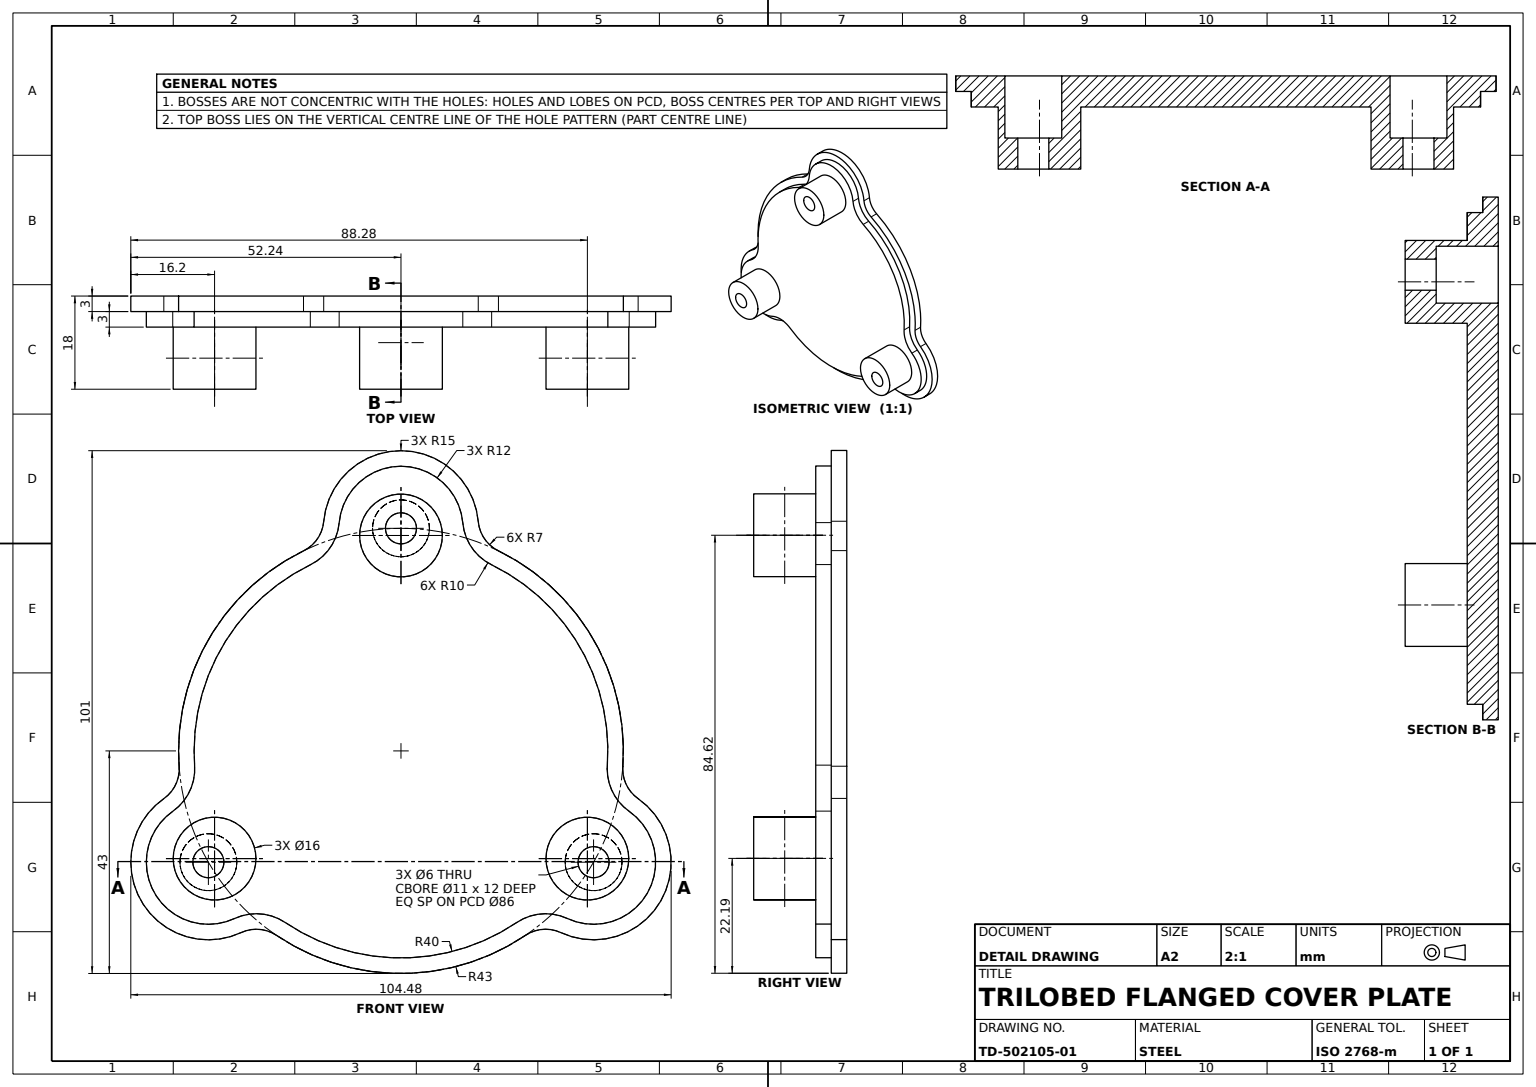
ISO-10303-21;
HEADER;
FILE_DESCRIPTION((''),'2;1');
FILE_NAME('','',(''),(''),'','','');
FILE_SCHEMA(('AUTOMOTIVE_DESIGN'));
ENDSEC;
DATA;
#1=APPLICATION_CONTEXT('');
#2=PRODUCT_CONTEXT('',#1,'mechanical');
#3=PRODUCT('','','',(#2));
#4=PRODUCT_DEFINITION_FORMATION('','',#3);
#5=PRODUCT_DEFINITION_CONTEXT('',#1,'design');
#6=PRODUCT_DEFINITION('','',#4,#5);
#7=PRODUCT_DEFINITION_SHAPE('','',#6);
#8=(LENGTH_UNIT()NAMED_UNIT(*)SI_UNIT(.MILLI.,.METRE.));
#9=(NAMED_UNIT(*)PLANE_ANGLE_UNIT()SI_UNIT($,.RADIAN.));
#10=(NAMED_UNIT(*)SI_UNIT($,.STERADIAN.)SOLID_ANGLE_UNIT());
#11=UNCERTAINTY_MEASURE_WITH_UNIT(LENGTH_MEASURE(1.E-05),#8,'distance_accuracy_value','');
#12=(GEOMETRIC_REPRESENTATION_CONTEXT(3)GLOBAL_UNCERTAINTY_ASSIGNED_CONTEXT((#11))GLOBAL_UNIT_ASSIGNED_CONTEXT((#8,#9,#10))REPRESENTATION_CONTEXT('',''));
#13=CARTESIAN_POINT('',(24.048805,-35.646248,-3.));
#14=VERTEX_POINT('',#13);
#15=CARTESIAN_POINT('',(24.048805,-35.646248,0.));
#16=VERTEX_POINT('',#15);
#17=DIRECTION('',(0.,0.,1.));
#18=VECTOR('',#17,1000.);
#19=LINE('',#13,#18);
#20=EDGE_CURVE('',#14,#16,#19,.T.);
#21=ORIENTED_EDGE('',*,*,#20,.T.);
#22=CARTESIAN_POINT('',(-24.048805,-35.646248,0.));
#23=VERTEX_POINT('',#22);
#24=CARTESIAN_POINT('',(0.,0.,0.));
#25=DIRECTION('',(1.,0.,0.));
#26=AXIS2_PLACEMENT_3D('',#24,#17,#25);
#27=CIRCLE('',#26,43.);
#28=EDGE_CURVE('',#23,#16,#27,.T.);
#29=ORIENTED_EDGE('',*,*,#28,.F.);
#30=CARTESIAN_POINT('',(-24.048805,-35.646248,-3.));
#31=VERTEX_POINT('',#30);
#32=LINE('',#30,#18);
#33=EDGE_CURVE('',#31,#23,#32,.T.);
#34=ORIENTED_EDGE('',*,*,#33,.F.);
#35=CARTESIAN_POINT('',(0.,0.,-3.));
#36=AXIS2_PLACEMENT_3D('',#35,#17,#25);
#37=CIRCLE('',#36,43.);
#38=EDGE_CURVE('',#31,#14,#37,.T.);
#39=ORIENTED_EDGE('',*,*,#38,.T.);
#40=EDGE_LOOP('',(#21,#29,#34,#39));
#41=FACE_OUTER_BOUND('',#40,.T.);
#42=CYLINDRICAL_SURFACE('',#36,43.);
#43=ADVANCED_FACE('',(#41),#42,.T.);
#44=CARTESIAN_POINT('',(-28.042979,-20.809424,-18.));
#45=VERTEX_POINT('',#44);
#46=CARTESIAN_POINT('',(-44.042979,-20.809424,-18.));
#47=VERTEX_POINT('',#46);
#48=CARTESIAN_POINT('',(-36.042979,-20.809424,-18.));
#49=DIRECTION('',(0.,0.,-1.));
#50=DIRECTION('',(-1.,0.,0.));
#51=AXIS2_PLACEMENT_3D('',#48,#49,#50);
#52=CIRCLE('',#51,8.);
#53=EDGE_CURVE('',#45,#47,#52,.T.);
#54=ORIENTED_EDGE('',*,*,#53,.T.);
#55=EDGE_CURVE('',#47,#45,#52,.T.);
#56=ORIENTED_EDGE('',*,*,#55,.T.);
#57=EDGE_LOOP('',(#54,#56));
#58=FACE_OUTER_BOUND('',#57,.T.);
#59=CARTESIAN_POINT('',(-34.239092,-21.5,-18.));
#60=VERTEX_POINT('',#59);
#61=CARTESIAN_POINT('',(-40.239092,-21.5,-18.));
#62=VERTEX_POINT('',#61);
#63=CARTESIAN_POINT('',(-37.239092,-21.5,-18.));
#64=AXIS2_PLACEMENT_3D('',#63,#49,#50);
#65=CIRCLE('',#64,3.);
#66=EDGE_CURVE('',#60,#62,#65,.T.);
#67=ORIENTED_EDGE('',*,*,#66,.F.);
#68=EDGE_CURVE('',#62,#60,#65,.T.);
#69=ORIENTED_EDGE('',*,*,#68,.F.);
#70=EDGE_LOOP('',(#67,#69));
#71=FACE_BOUND('',#70,.T.);
#72=PLANE('',#51);
#73=ADVANCED_FACE('',(#58,#71),#72,.T.);
#74=CARTESIAN_POINT('',(-44.042979,-20.809424,-6.));
#75=VERTEX_POINT('',#74);
#76=CARTESIAN_POINT('',(-28.042979,-20.809424,-6.));
#77=VERTEX_POINT('',#76);
#78=CARTESIAN_POINT('',(-36.042979,-20.809424,-6.));
#79=AXIS2_PLACEMENT_3D('',#78,#49,#50);
#80=CIRCLE('',#79,8.);
#81=EDGE_CURVE('',#75,#77,#80,.T.);
#82=ORIENTED_EDGE('',*,*,#81,.T.);
#83=LINE('',#44,#18);
#84=EDGE_CURVE('',#45,#77,#83,.T.);
#85=ORIENTED_EDGE('',*,*,#84,.F.);
#86=ORIENTED_EDGE('',*,*,#55,.F.);
#87=LINE('',#46,#18);
#88=EDGE_CURVE('',#47,#75,#87,.T.);
#89=ORIENTED_EDGE('',*,*,#88,.T.);
#90=EDGE_LOOP('',(#82,#85,#86,#89));
#91=FACE_OUTER_BOUND('',#90,.T.);
#92=AXIS2_PLACEMENT_3D('',#48,#17,#25);
#93=CYLINDRICAL_SURFACE('',#92,8.);
#94=ADVANCED_FACE('',(#91),#93,.T.);
#95=CARTESIAN_POINT('',(22.370982,-33.1593,-6.));
#96=VERTEX_POINT('',#95);
#97=CARTESIAN_POINT('',(-22.370982,-33.1593,-6.));
#98=VERTEX_POINT('',#97);
#99=CARTESIAN_POINT('',(0.,0.,-6.));
#100=AXIS2_PLACEMENT_3D('',#99,#49,#50);
#101=CIRCLE('',#100,40.);
#102=EDGE_CURVE('',#96,#98,#101,.T.);
#103=ORIENTED_EDGE('',*,*,#102,.T.);
#104=CARTESIAN_POINT('',(-32.179802,-32.381341,-6.));
#105=VERTEX_POINT('',#104);
#106=CARTESIAN_POINT('',(-27.963727,-41.449125,-6.));
#107=AXIS2_PLACEMENT_3D('',#106,#17,#50);
#108=CIRCLE('',#107,10.);
#109=EDGE_CURVE('',#98,#105,#108,.T.);
#110=ORIENTED_EDGE('',*,*,#109,.T.);
#111=CARTESIAN_POINT('',(-44.132965,-11.677856,-6.));
#112=VERTEX_POINT('',#111);
#113=CARTESIAN_POINT('',(-37.239092,-21.5,-6.));
#114=AXIS2_PLACEMENT_3D('',#113,#49,#50);
#115=CIRCLE('',#114,12.);
#116=EDGE_CURVE('',#105,#112,#115,.T.);
#117=ORIENTED_EDGE('',*,*,#116,.T.);
#118=CARTESIAN_POINT('',(-39.877859,-3.492735,-6.));
#119=VERTEX_POINT('',#118);
#120=CARTESIAN_POINT('',(-49.877859,-3.492735,-6.));
#121=AXIS2_PLACEMENT_3D('',#120,#17,#50);
#122=CIRCLE('',#121,10.);
#123=EDGE_CURVE('',#112,#119,#122,.T.);
#124=ORIENTED_EDGE('',*,*,#123,.T.);
#125=CARTESIAN_POINT('',(-39.902287,-2.794188,-6.));
#126=VERTEX_POINT('',#125);
#127=EDGE_CURVE('',#119,#126,#122,.T.);
#128=ORIENTED_EDGE('',*,*,#127,.T.);
#129=CARTESIAN_POINT('',(-17.531306,35.953488,-6.));
#130=VERTEX_POINT('',#129);
#131=EDGE_CURVE('',#126,#130,#101,.T.);
#132=ORIENTED_EDGE('',*,*,#131,.T.);
#133=CARTESIAN_POINT('',(-11.953163,44.059197,-6.));
#134=VERTEX_POINT('',#133);
#135=CARTESIAN_POINT('',(-21.914132,44.94186,-6.));
#136=AXIS2_PLACEMENT_3D('',#135,#17,#50);
#137=CIRCLE('',#136,10.);
#138=EDGE_CURVE('',#130,#134,#137,.T.);
#139=ORIENTED_EDGE('',*,*,#138,.T.);
#140=CARTESIAN_POINT('',(11.953163,44.059197,-6.));
#141=VERTEX_POINT('',#140);
#142=CARTESIAN_POINT('',(0.,43.,-6.));
#143=AXIS2_PLACEMENT_3D('',#142,#49,#50);
#144=CIRCLE('',#143,12.);
#145=EDGE_CURVE('',#134,#141,#144,.T.);
#146=ORIENTED_EDGE('',*,*,#145,.T.);
#147=CARTESIAN_POINT('',(17.531306,35.953488,-6.));
#148=VERTEX_POINT('',#147);
#149=CARTESIAN_POINT('',(21.914132,44.94186,-6.));
#150=AXIS2_PLACEMENT_3D('',#149,#17,#50);
#151=CIRCLE('',#150,10.);
#152=EDGE_CURVE('',#141,#148,#151,.T.);
#153=ORIENTED_EDGE('',*,*,#152,.T.);
#154=CARTESIAN_POINT('',(40.,0.,-6.));
#155=VERTEX_POINT('',#154);
#156=EDGE_CURVE('',#148,#155,#101,.T.);
#157=ORIENTED_EDGE('',*,*,#156,.T.);
#158=CARTESIAN_POINT('',(39.902287,-2.794188,-6.));
#159=VERTEX_POINT('',#158);
#160=EDGE_CURVE('',#155,#159,#101,.T.);
#161=ORIENTED_EDGE('',*,*,#160,.T.);
#162=CARTESIAN_POINT('',(44.132965,-11.677856,-6.));
#163=VERTEX_POINT('',#162);
#164=CARTESIAN_POINT('',(49.877859,-3.492735,-6.));
#165=AXIS2_PLACEMENT_3D('',#164,#17,#50);
#166=CIRCLE('',#165,10.);
#167=EDGE_CURVE('',#159,#163,#166,.T.);
#168=ORIENTED_EDGE('',*,*,#167,.T.);
#169=CARTESIAN_POINT('',(49.239092,-21.5,-6.));
#170=VERTEX_POINT('',#169);
#171=CARTESIAN_POINT('',(37.239092,-21.5,-6.));
#172=AXIS2_PLACEMENT_3D('',#171,#49,#50);
#173=CIRCLE('',#172,12.);
#174=EDGE_CURVE('',#163,#170,#173,.T.);
#175=ORIENTED_EDGE('',*,*,#174,.T.);
#176=CARTESIAN_POINT('',(32.179802,-32.381341,-6.));
#177=VERTEX_POINT('',#176);
#178=EDGE_CURVE('',#170,#177,#173,.T.);
#179=ORIENTED_EDGE('',*,*,#178,.T.);
#180=CARTESIAN_POINT('',(27.963727,-41.449125,-6.));
#181=AXIS2_PLACEMENT_3D('',#180,#17,#50);
#182=CIRCLE('',#181,10.);
#183=EDGE_CURVE('',#177,#96,#182,.T.);
#184=ORIENTED_EDGE('',*,*,#183,.T.);
#185=EDGE_LOOP('',(#103,#110,#117,#124,#128,#132,#139,#146,#153,#157,#161,#168,#175,#179,#184));
#186=FACE_OUTER_BOUND('',#185,.T.);
#187=CARTESIAN_POINT('',(44.042979,-20.809424,-6.));
#188=VERTEX_POINT('',#187);
#189=CARTESIAN_POINT('',(28.042979,-20.809424,-6.));
#190=VERTEX_POINT('',#189);
#191=CARTESIAN_POINT('',(36.042979,-20.809424,-6.));
#192=AXIS2_PLACEMENT_3D('',#191,#49,#50);
#193=CIRCLE('',#192,8.);
#194=EDGE_CURVE('',#188,#190,#193,.T.);
#195=ORIENTED_EDGE('',*,*,#194,.F.);
#196=EDGE_CURVE('',#190,#188,#193,.T.);
#197=ORIENTED_EDGE('',*,*,#196,.F.);
#198=EDGE_LOOP('',(#195,#197));
#199=FACE_BOUND('',#198,.T.);
#200=CARTESIAN_POINT('',(8.,41.618847,-6.));
#201=VERTEX_POINT('',#200);
#202=CARTESIAN_POINT('',(-8.,41.618847,-6.));
#203=VERTEX_POINT('',#202);
#204=CARTESIAN_POINT('',(0.,41.618847,-6.));
#205=AXIS2_PLACEMENT_3D('',#204,#49,#50);
#206=CIRCLE('',#205,8.);
#207=EDGE_CURVE('',#201,#203,#206,.T.);
#208=ORIENTED_EDGE('',*,*,#207,.F.);
#209=EDGE_CURVE('',#203,#201,#206,.T.);
#210=ORIENTED_EDGE('',*,*,#209,.F.);
#211=EDGE_LOOP('',(#208,#210));
#212=FACE_BOUND('',#211,.T.);
#213=ORIENTED_EDGE('',*,*,#81,.F.);
#214=EDGE_CURVE('',#77,#75,#80,.T.);
#215=ORIENTED_EDGE('',*,*,#214,.F.);
#216=EDGE_LOOP('',(#213,#215));
#217=FACE_BOUND('',#216,.T.);
#218=CARTESIAN_POINT('',(10.957066,43.97093,-6.));
#219=AXIS2_PLACEMENT_3D('',#218,#49,#50);
#220=PLANE('',#219);
#221=ADVANCED_FACE('',(#186,#199,#212,#217),#220,.T.);
#222=CARTESIAN_POINT('',(-8.,41.618847,-18.));
#223=VERTEX_POINT('',#222);
#224=CARTESIAN_POINT('',(8.,41.618847,-18.));
#225=VERTEX_POINT('',#224);
#226=CARTESIAN_POINT('',(0.,41.618847,-18.));
#227=AXIS2_PLACEMENT_3D('',#226,#49,#50);
#228=CIRCLE('',#227,8.);
#229=EDGE_CURVE('',#223,#225,#228,.T.);
#230=ORIENTED_EDGE('',*,*,#229,.F.);
#231=LINE('',#222,#18);
#232=EDGE_CURVE('',#223,#203,#231,.T.);
#233=ORIENTED_EDGE('',*,*,#232,.T.);
#234=ORIENTED_EDGE('',*,*,#209,.T.);
#235=LINE('',#224,#18);
#236=EDGE_CURVE('',#225,#201,#235,.T.);
#237=ORIENTED_EDGE('',*,*,#236,.F.);
#238=EDGE_LOOP('',(#230,#233,#234,#237));
#239=FACE_OUTER_BOUND('',#238,.T.);
#240=AXIS2_PLACEMENT_3D('',#226,#17,#25);
#241=CYLINDRICAL_SURFACE('',#240,8.);
#242=ADVANCED_FACE('',(#239),#241,.T.);
#243=CARTESIAN_POINT('',(-30.91498,-35.101676,-3.));
#244=VERTEX_POINT('',#243);
#245=CARTESIAN_POINT('',(-30.91498,-35.101676,0.));
#246=VERTEX_POINT('',#245);
#247=LINE('',#243,#18);
#248=EDGE_CURVE('',#244,#246,#247,.T.);
#249=ORIENTED_EDGE('',*,*,#248,.F.);
#250=CARTESIAN_POINT('',(-27.963727,-41.449125,-3.));
#251=AXIS2_PLACEMENT_3D('',#250,#49,#50);
#252=CIRCLE('',#251,7.);
#253=EDGE_CURVE('',#244,#31,#252,.T.);
#254=ORIENTED_EDGE('',*,*,#253,.T.);
#255=ORIENTED_EDGE('',*,*,#33,.T.);
#256=CARTESIAN_POINT('',(-27.963727,-41.449125,0.));
#257=AXIS2_PLACEMENT_3D('',#256,#49,#50);
#258=CIRCLE('',#257,7.);
#259=EDGE_CURVE('',#246,#23,#258,.T.);
#260=ORIENTED_EDGE('',*,*,#259,.F.);
#261=EDGE_LOOP('',(#249,#254,#255,#260));
#262=FACE_OUTER_BOUND('',#261,.T.);
#263=AXIS2_PLACEMENT_3D('',#250,#17,#25);
#264=CYLINDRICAL_SURFACE('',#263,7.);
#265=ADVANCED_FACE('',(#262),#264,.F.);
#266=CARTESIAN_POINT('',(-5.5,43.,-12.));
#267=VERTEX_POINT('',#266);
#268=CARTESIAN_POINT('',(5.5,43.,-12.));
#269=VERTEX_POINT('',#268);
#270=CARTESIAN_POINT('',(0.,43.,-12.));
#271=AXIS2_PLACEMENT_3D('',#270,#17,#25);
#272=CIRCLE('',#271,5.5);
#273=EDGE_CURVE('',#267,#269,#272,.T.);
#274=ORIENTED_EDGE('',*,*,#273,.F.);
#275=CARTESIAN_POINT('',(-5.5,43.,0.));
#276=VERTEX_POINT('',#275);
#277=LINE('',#266,#18);
#278=EDGE_CURVE('',#267,#276,#277,.T.);
#279=ORIENTED_EDGE('',*,*,#278,.T.);
#280=CARTESIAN_POINT('',(5.5,43.,0.));
#281=VERTEX_POINT('',#280);
#282=CARTESIAN_POINT('',(0.,43.,0.));
#283=AXIS2_PLACEMENT_3D('',#282,#17,#25);
#284=CIRCLE('',#283,5.5);
#285=EDGE_CURVE('',#276,#281,#284,.T.);
#286=ORIENTED_EDGE('',*,*,#285,.T.);
#287=LINE('',#268,#18);
#288=EDGE_CURVE('',#269,#281,#287,.T.);
#289=ORIENTED_EDGE('',*,*,#288,.F.);
#290=EDGE_LOOP('',(#274,#279,#286,#289));
#291=FACE_OUTER_BOUND('',#290,.T.);
#292=CYLINDRICAL_SURFACE('',#271,5.5);
#293=ADVANCED_FACE('',(#291),#292,.F.);
#294=ORIENTED_EDGE('',*,*,#288,.T.);
#295=EDGE_CURVE('',#281,#276,#284,.T.);
#296=ORIENTED_EDGE('',*,*,#295,.T.);
#297=ORIENTED_EDGE('',*,*,#278,.F.);
#298=EDGE_CURVE('',#269,#267,#272,.T.);
#299=ORIENTED_EDGE('',*,*,#298,.F.);
#300=EDGE_LOOP('',(#294,#296,#297,#299));
#301=FACE_OUTER_BOUND('',#300,.T.);
#302=ADVANCED_FACE('',(#301),#292,.F.);
#303=CARTESIAN_POINT('',(-42.739092,-21.5,-12.));
#304=VERTEX_POINT('',#303);
#305=CARTESIAN_POINT('',(-42.739092,-21.5,0.));
#306=VERTEX_POINT('',#305);
#307=LINE('',#303,#18);
#308=EDGE_CURVE('',#304,#306,#307,.T.);
#309=ORIENTED_EDGE('',*,*,#308,.T.);
#310=CARTESIAN_POINT('',(-31.739092,-21.5,0.));
#311=VERTEX_POINT('',#310);
#312=CARTESIAN_POINT('',(-37.239092,-21.5,0.));
#313=AXIS2_PLACEMENT_3D('',#312,#17,#25);
#314=CIRCLE('',#313,5.5);
#315=EDGE_CURVE('',#306,#311,#314,.T.);
#316=ORIENTED_EDGE('',*,*,#315,.T.);
#317=CARTESIAN_POINT('',(-31.739092,-21.5,-12.));
#318=VERTEX_POINT('',#317);
#319=LINE('',#317,#18);
#320=EDGE_CURVE('',#318,#311,#319,.T.);
#321=ORIENTED_EDGE('',*,*,#320,.F.);
#322=CARTESIAN_POINT('',(-37.239092,-21.5,-12.));
#323=AXIS2_PLACEMENT_3D('',#322,#17,#25);
#324=CIRCLE('',#323,5.5);
#325=EDGE_CURVE('',#304,#318,#324,.T.);
#326=ORIENTED_EDGE('',*,*,#325,.F.);
#327=EDGE_LOOP('',(#309,#316,#321,#326));
#328=FACE_OUTER_BOUND('',#327,.T.);
#329=CYLINDRICAL_SURFACE('',#323,5.5);
#330=ADVANCED_FACE('',(#328),#329,.F.);
#331=CARTESIAN_POINT('',(-17.531306,35.953488,-3.));
#332=VERTEX_POINT('',#331);
#333=LINE('',#129,#18);
#334=EDGE_CURVE('',#130,#332,#333,.T.);
#335=ORIENTED_EDGE('',*,*,#334,.T.);
#336=CARTESIAN_POINT('',(-11.953163,44.059197,-3.));
#337=VERTEX_POINT('',#336);
#338=CARTESIAN_POINT('',(-21.914132,44.94186,-3.));
#339=AXIS2_PLACEMENT_3D('',#338,#17,#50);
#340=CIRCLE('',#339,10.);
#341=EDGE_CURVE('',#332,#337,#340,.T.);
#342=ORIENTED_EDGE('',*,*,#341,.T.);
#343=LINE('',#133,#18);
#344=EDGE_CURVE('',#134,#337,#343,.T.);
#345=ORIENTED_EDGE('',*,*,#344,.F.);
#346=ORIENTED_EDGE('',*,*,#138,.F.);
#347=EDGE_LOOP('',(#335,#342,#345,#346));
#348=FACE_OUTER_BOUND('',#347,.T.);
#349=AXIS2_PLACEMENT_3D('',#135,#17,#25);
#350=CYLINDRICAL_SURFACE('',#349,10.);
#351=ADVANCED_FACE('',(#348),#350,.F.);
#352=CARTESIAN_POINT('',(-44.132965,-11.677856,-3.));
#353=VERTEX_POINT('',#352);
#354=CARTESIAN_POINT('',(-39.877859,-3.492735,-3.));
#355=VERTEX_POINT('',#354);
#356=CARTESIAN_POINT('',(-49.877859,-3.492735,-3.));
#357=AXIS2_PLACEMENT_3D('',#356,#17,#50);
#358=CIRCLE('',#357,10.);
#359=EDGE_CURVE('',#353,#355,#358,.T.);
#360=ORIENTED_EDGE('',*,*,#359,.T.);
#361=LINE('',#118,#18);
#362=EDGE_CURVE('',#119,#355,#361,.T.);
#363=ORIENTED_EDGE('',*,*,#362,.F.);
#364=ORIENTED_EDGE('',*,*,#123,.F.);
#365=LINE('',#111,#18);
#366=EDGE_CURVE('',#112,#353,#365,.T.);
#367=ORIENTED_EDGE('',*,*,#366,.T.);
#368=EDGE_LOOP('',(#360,#363,#364,#367));
#369=FACE_OUTER_BOUND('',#368,.T.);
#370=AXIS2_PLACEMENT_3D('',#120,#17,#25);
#371=CYLINDRICAL_SURFACE('',#370,10.);
#372=ADVANCED_FACE('',(#369),#371,.F.);
#373=CARTESIAN_POINT('',(17.531306,35.953488,-3.));
#374=VERTEX_POINT('',#373);
#375=CARTESIAN_POINT('',(40.,0.,-3.));
#376=VERTEX_POINT('',#375);
#377=AXIS2_PLACEMENT_3D('',#35,#49,#50);
#378=CIRCLE('',#377,40.);
#379=EDGE_CURVE('',#374,#376,#378,.T.);
#380=ORIENTED_EDGE('',*,*,#379,.T.);
#381=LINE('',#154,#18);
#382=EDGE_CURVE('',#155,#376,#381,.T.);
#383=ORIENTED_EDGE('',*,*,#382,.F.);
#384=ORIENTED_EDGE('',*,*,#156,.F.);
#385=LINE('',#147,#18);
#386=EDGE_CURVE('',#148,#374,#385,.T.);
#387=ORIENTED_EDGE('',*,*,#386,.T.);
#388=EDGE_LOOP('',(#380,#383,#384,#387));
#389=FACE_OUTER_BOUND('',#388,.T.);
#390=AXIS2_PLACEMENT_3D('',#99,#17,#25);
#391=CYLINDRICAL_SURFACE('',#390,40.);
#392=ADVANCED_FACE('',(#389),#391,.T.);
#393=CARTESIAN_POINT('',(-42.894959,-3.003752,-3.));
#394=VERTEX_POINT('',#393);
#395=CARTESIAN_POINT('',(-42.877859,-3.492735,-3.));
#396=VERTEX_POINT('',#395);
#397=AXIS2_PLACEMENT_3D('',#356,#49,#25);
#398=CIRCLE('',#397,7.);
#399=EDGE_CURVE('',#394,#396,#398,.T.);
#400=ORIENTED_EDGE('',*,*,#399,.T.);
#401=CARTESIAN_POINT('',(-42.877859,-3.492735,0.));
#402=VERTEX_POINT('',#401);
#403=LINE('',#395,#18);
#404=EDGE_CURVE('',#396,#402,#403,.T.);
#405=ORIENTED_EDGE('',*,*,#404,.T.);
#406=CARTESIAN_POINT('',(-42.894959,-3.003752,0.));
#407=VERTEX_POINT('',#406);
#408=CARTESIAN_POINT('',(-49.877859,-3.492735,0.));
#409=AXIS2_PLACEMENT_3D('',#408,#49,#25);
#410=CIRCLE('',#409,7.);
#411=EDGE_CURVE('',#407,#402,#410,.T.);
#412=ORIENTED_EDGE('',*,*,#411,.F.);
#413=LINE('',#393,#18);
#414=EDGE_CURVE('',#394,#407,#413,.T.);
#415=ORIENTED_EDGE('',*,*,#414,.F.);
#416=EDGE_LOOP('',(#400,#405,#412,#415));
#417=FACE_OUTER_BOUND('',#416,.T.);
#418=AXIS2_PLACEMENT_3D('',#356,#17,#25);
#419=CYLINDRICAL_SURFACE('',#418,7.);
#420=ADVANCED_FACE('',(#417),#419,.F.);
#421=ORIENTED_EDGE('',*,*,#183,.F.);
#422=CARTESIAN_POINT('',(32.179802,-32.381341,-3.));
#423=VERTEX_POINT('',#422);
#424=LINE('',#176,#18);
#425=EDGE_CURVE('',#177,#423,#424,.T.);
#426=ORIENTED_EDGE('',*,*,#425,.T.);
#427=CARTESIAN_POINT('',(22.370982,-33.1593,-3.));
#428=VERTEX_POINT('',#427);
#429=CARTESIAN_POINT('',(27.963727,-41.449125,-3.));
#430=AXIS2_PLACEMENT_3D('',#429,#17,#50);
#431=CIRCLE('',#430,10.);
#432=EDGE_CURVE('',#423,#428,#431,.T.);
#433=ORIENTED_EDGE('',*,*,#432,.T.);
#434=LINE('',#95,#18);
#435=EDGE_CURVE('',#96,#428,#434,.T.);
#436=ORIENTED_EDGE('',*,*,#435,.F.);
#437=EDGE_LOOP('',(#421,#426,#433,#436));
#438=FACE_OUTER_BOUND('',#437,.T.);
#439=AXIS2_PLACEMENT_3D('',#180,#17,#25);
#440=CYLINDRICAL_SURFACE('',#439,10.);
#441=ADVANCED_FACE('',(#438),#440,.F.);
#442=CARTESIAN_POINT('',(-3.,43.,-18.));
#443=VERTEX_POINT('',#442);
#444=CARTESIAN_POINT('',(3.,43.,-18.));
#445=VERTEX_POINT('',#444);
#446=CARTESIAN_POINT('',(0.,43.,-18.));
#447=AXIS2_PLACEMENT_3D('',#446,#49,#50);
#448=CIRCLE('',#447,3.);
#449=EDGE_CURVE('',#443,#445,#448,.T.);
#450=ORIENTED_EDGE('',*,*,#449,.F.);
#451=EDGE_CURVE('',#445,#443,#448,.T.);
#452=ORIENTED_EDGE('',*,*,#451,.F.);
#453=EDGE_LOOP('',(#450,#452));
#454=FACE_BOUND('',#453,.T.);
#455=ORIENTED_EDGE('',*,*,#229,.T.);
#456=EDGE_CURVE('',#225,#223,#228,.T.);
#457=ORIENTED_EDGE('',*,*,#456,.T.);
#458=EDGE_LOOP('',(#455,#457));
#459=FACE_OUTER_BOUND('',#458,.T.);
#460=PLANE('',#227);
#461=ADVANCED_FACE('',(#454,#459),#460,.T.);
#462=CARTESIAN_POINT('',(40.239092,-21.5,-18.));
#463=VERTEX_POINT('',#462);
#464=CARTESIAN_POINT('',(34.239092,-21.5,-18.));
#465=VERTEX_POINT('',#464);
#466=CARTESIAN_POINT('',(37.239092,-21.5,-18.));
#467=AXIS2_PLACEMENT_3D('',#466,#49,#50);
#468=CIRCLE('',#467,3.);
#469=EDGE_CURVE('',#463,#465,#468,.T.);
#470=ORIENTED_EDGE('',*,*,#469,.F.);
#471=EDGE_CURVE('',#465,#463,#468,.T.);
#472=ORIENTED_EDGE('',*,*,#471,.F.);
#473=EDGE_LOOP('',(#470,#472));
#474=FACE_BOUND('',#473,.T.);
#475=CARTESIAN_POINT('',(28.042979,-20.809424,-18.));
#476=VERTEX_POINT('',#475);
#477=CARTESIAN_POINT('',(44.042979,-20.809424,-18.));
#478=VERTEX_POINT('',#477);
#479=CARTESIAN_POINT('',(36.042979,-20.809424,-18.));
#480=AXIS2_PLACEMENT_3D('',#479,#49,#50);
#481=CIRCLE('',#480,8.);
#482=EDGE_CURVE('',#476,#478,#481,.T.);
#483=ORIENTED_EDGE('',*,*,#482,.T.);
#484=EDGE_CURVE('',#478,#476,#481,.T.);
#485=ORIENTED_EDGE('',*,*,#484,.T.);
#486=EDGE_LOOP('',(#483,#485));
#487=FACE_OUTER_BOUND('',#486,.T.);
#488=PLANE('',#480);
#489=ADVANCED_FACE('',(#474,#487),#488,.T.);
#490=CARTESIAN_POINT('',(45.856433,-9.22232,-3.));
#491=VERTEX_POINT('',#490);
#492=CARTESIAN_POINT('',(45.856433,-9.22232,0.));
#493=VERTEX_POINT('',#492);
#494=LINE('',#490,#18);
#495=EDGE_CURVE('',#491,#493,#494,.T.);
#496=ORIENTED_EDGE('',*,*,#495,.T.);
#497=CARTESIAN_POINT('',(52.239092,-21.5,0.));
#498=VERTEX_POINT('',#497);
#499=CARTESIAN_POINT('',(37.239092,-21.5,0.));
#500=AXIS2_PLACEMENT_3D('',#499,#17,#25);
#501=CIRCLE('',#500,15.);
#502=EDGE_CURVE('',#498,#493,#501,.T.);
#503=ORIENTED_EDGE('',*,*,#502,.F.);
#504=CARTESIAN_POINT('',(52.239092,-21.5,-3.));
#505=VERTEX_POINT('',#504);
#506=LINE('',#504,#18);
#507=EDGE_CURVE('',#505,#498,#506,.T.);
#508=ORIENTED_EDGE('',*,*,#507,.F.);
#509=CARTESIAN_POINT('',(37.239092,-21.5,-3.));
#510=AXIS2_PLACEMENT_3D('',#509,#17,#25);
#511=CIRCLE('',#510,15.);
#512=EDGE_CURVE('',#505,#491,#511,.T.);
#513=ORIENTED_EDGE('',*,*,#512,.T.);
#514=EDGE_LOOP('',(#496,#503,#508,#513));
#515=FACE_OUTER_BOUND('',#514,.T.);
#516=CYLINDRICAL_SURFACE('',#510,15.);
#517=ADVANCED_FACE('',(#515),#516,.T.);
#518=CARTESIAN_POINT('',(-45.856433,-9.22232,0.));
#519=VERTEX_POINT('',#518);
#520=EDGE_CURVE('',#402,#519,#410,.T.);
#521=ORIENTED_EDGE('',*,*,#520,.F.);
#522=ORIENTED_EDGE('',*,*,#404,.F.);
#523=CARTESIAN_POINT('',(-45.856433,-9.22232,-3.));
#524=VERTEX_POINT('',#523);
#525=EDGE_CURVE('',#396,#524,#398,.T.);
#526=ORIENTED_EDGE('',*,*,#525,.T.);
#527=LINE('',#523,#18);
#528=EDGE_CURVE('',#524,#519,#527,.T.);
#529=ORIENTED_EDGE('',*,*,#528,.T.);
#530=EDGE_LOOP('',(#521,#522,#526,#529));
#531=FACE_OUTER_BOUND('',#530,.T.);
#532=ADVANCED_FACE('',(#531),#419,.F.);
#533=CARTESIAN_POINT('',(31.739092,-21.5,0.));
#534=VERTEX_POINT('',#533);
#535=CARTESIAN_POINT('',(42.739092,-21.5,0.));
#536=VERTEX_POINT('',#535);
#537=CIRCLE('',#500,5.5);
#538=EDGE_CURVE('',#534,#536,#537,.T.);
#539=ORIENTED_EDGE('',*,*,#538,.T.);
#540=CARTESIAN_POINT('',(42.739092,-21.5,-12.));
#541=VERTEX_POINT('',#540);
#542=LINE('',#540,#18);
#543=EDGE_CURVE('',#541,#536,#542,.T.);
#544=ORIENTED_EDGE('',*,*,#543,.F.);
#545=CARTESIAN_POINT('',(31.739092,-21.5,-12.));
#546=VERTEX_POINT('',#545);
#547=CARTESIAN_POINT('',(37.239092,-21.5,-12.));
#548=AXIS2_PLACEMENT_3D('',#547,#17,#25);
#549=CIRCLE('',#548,5.5);
#550=EDGE_CURVE('',#546,#541,#549,.T.);
#551=ORIENTED_EDGE('',*,*,#550,.F.);
#552=LINE('',#545,#18);
#553=EDGE_CURVE('',#546,#534,#552,.T.);
#554=ORIENTED_EDGE('',*,*,#553,.T.);
#555=EDGE_LOOP('',(#539,#544,#551,#554));
#556=FACE_OUTER_BOUND('',#555,.T.);
#557=CYLINDRICAL_SURFACE('',#548,5.5);
#558=ADVANCED_FACE('',(#556),#557,.F.);
#559=ORIENTED_EDGE('',*,*,#207,.T.);
#560=ORIENTED_EDGE('',*,*,#232,.F.);
#561=ORIENTED_EDGE('',*,*,#456,.F.);
#562=ORIENTED_EDGE('',*,*,#236,.T.);
#563=EDGE_LOOP('',(#559,#560,#561,#562));
#564=FACE_OUTER_BOUND('',#563,.T.);
#565=ADVANCED_FACE('',(#564),#241,.T.);
#566=CARTESIAN_POINT('',(-3.,43.,-12.));
#567=VERTEX_POINT('',#566);
#568=CARTESIAN_POINT('',(3.,43.,-12.));
#569=VERTEX_POINT('',#568);
#570=CIRCLE('',#271,3.);
#571=EDGE_CURVE('',#567,#569,#570,.T.);
#572=ORIENTED_EDGE('',*,*,#571,.F.);
#573=EDGE_CURVE('',#569,#567,#570,.T.);
#574=ORIENTED_EDGE('',*,*,#573,.F.);
#575=EDGE_LOOP('',(#572,#574));
#576=FACE_BOUND('',#575,.T.);
#577=ORIENTED_EDGE('',*,*,#273,.T.);
#578=ORIENTED_EDGE('',*,*,#298,.T.);
#579=EDGE_LOOP('',(#577,#578));
#580=FACE_OUTER_BOUND('',#579,.T.);
#581=PLANE('',#271);
#582=ADVANCED_FACE('',(#576,#580),#581,.T.);
#583=ORIENTED_EDGE('',*,*,#382,.T.);
#584=CARTESIAN_POINT('',(39.902287,-2.794188,-3.));
#585=VERTEX_POINT('',#584);
#586=EDGE_CURVE('',#376,#585,#378,.T.);
#587=ORIENTED_EDGE('',*,*,#586,.T.);
#588=LINE('',#158,#18);
#589=EDGE_CURVE('',#159,#585,#588,.T.);
#590=ORIENTED_EDGE('',*,*,#589,.F.);
#591=ORIENTED_EDGE('',*,*,#160,.F.);
#592=EDGE_LOOP('',(#583,#587,#590,#591));
#593=FACE_OUTER_BOUND('',#592,.T.);
#594=ADVANCED_FACE('',(#593),#391,.T.);
#595=CARTESIAN_POINT('',(-37.239092,-21.5,-3.));
#596=AXIS2_PLACEMENT_3D('',#595,#17,#25);
#597=CIRCLE('',#596,15.);
#598=EDGE_CURVE('',#524,#244,#597,.T.);
#599=ORIENTED_EDGE('',*,*,#598,.T.);
#600=ORIENTED_EDGE('',*,*,#248,.T.);
#601=CIRCLE('',#313,15.);
#602=EDGE_CURVE('',#519,#246,#601,.T.);
#603=ORIENTED_EDGE('',*,*,#602,.F.);
#604=ORIENTED_EDGE('',*,*,#528,.F.);
#605=EDGE_LOOP('',(#599,#600,#603,#604));
#606=FACE_OUTER_BOUND('',#605,.T.);
#607=CYLINDRICAL_SURFACE('',#596,15.);
#608=ADVANCED_FACE('',(#606),#607,.T.);
#609=CARTESIAN_POINT('',(-22.370982,-33.1593,-3.));
#610=VERTEX_POINT('',#609);
#611=EDGE_CURVE('',#428,#610,#378,.T.);
#612=ORIENTED_EDGE('',*,*,#611,.T.);
#613=LINE('',#97,#18);
#614=EDGE_CURVE('',#98,#610,#613,.T.);
#615=ORIENTED_EDGE('',*,*,#614,.F.);
#616=ORIENTED_EDGE('',*,*,#102,.F.);
#617=ORIENTED_EDGE('',*,*,#435,.T.);
#618=EDGE_LOOP('',(#612,#615,#616,#617));
#619=FACE_OUTER_BOUND('',#618,.T.);
#620=ADVANCED_FACE('',(#619),#391,.T.);
#621=ORIENTED_EDGE('',*,*,#38,.F.);
#622=ORIENTED_EDGE('',*,*,#253,.F.);
#623=ORIENTED_EDGE('',*,*,#598,.F.);
#624=ORIENTED_EDGE('',*,*,#525,.F.);
#625=ORIENTED_EDGE('',*,*,#399,.F.);
#626=CARTESIAN_POINT('',(-18.846153,38.65,-3.));
#627=VERTEX_POINT('',#626);
#628=EDGE_CURVE('',#627,#394,#37,.T.);
#629=ORIENTED_EDGE('',*,*,#628,.F.);
#630=CARTESIAN_POINT('',(-14.941454,44.323996,-3.));
#631=VERTEX_POINT('',#630);
#632=AXIS2_PLACEMENT_3D('',#338,#49,#50);
#633=CIRCLE('',#632,7.);
#634=EDGE_CURVE('',#631,#627,#633,.T.);
#635=ORIENTED_EDGE('',*,*,#634,.F.);
#636=CARTESIAN_POINT('',(14.941454,44.323996,-3.));
#637=VERTEX_POINT('',#636);
#638=CARTESIAN_POINT('',(0.,43.,-3.));
#639=AXIS2_PLACEMENT_3D('',#638,#17,#25);
#640=CIRCLE('',#639,15.);
#641=EDGE_CURVE('',#637,#631,#640,.T.);
#642=ORIENTED_EDGE('',*,*,#641,.F.);
#643=CARTESIAN_POINT('',(18.846153,38.65,-3.));
#644=VERTEX_POINT('',#643);
#645=CARTESIAN_POINT('',(21.914132,44.94186,-3.));
#646=AXIS2_PLACEMENT_3D('',#645,#49,#25);
#647=CIRCLE('',#646,7.);
#648=EDGE_CURVE('',#644,#637,#647,.T.);
#649=ORIENTED_EDGE('',*,*,#648,.F.);
#650=CARTESIAN_POINT('',(43.,0.,-3.));
#651=VERTEX_POINT('',#650);
#652=EDGE_CURVE('',#651,#644,#37,.T.);
#653=ORIENTED_EDGE('',*,*,#652,.F.);
#654=CARTESIAN_POINT('',(42.894959,-3.003752,-3.));
#655=VERTEX_POINT('',#654);
#656=EDGE_CURVE('',#655,#651,#37,.T.);
#657=ORIENTED_EDGE('',*,*,#656,.F.);
#658=CARTESIAN_POINT('',(49.877859,-3.492735,-3.));
#659=AXIS2_PLACEMENT_3D('',#658,#49,#50);
#660=CIRCLE('',#659,7.);
#661=EDGE_CURVE('',#491,#655,#660,.T.);
#662=ORIENTED_EDGE('',*,*,#661,.F.);
#663=ORIENTED_EDGE('',*,*,#512,.F.);
#664=CARTESIAN_POINT('',(30.91498,-35.101676,-3.));
#665=VERTEX_POINT('',#664);
#666=EDGE_CURVE('',#665,#505,#511,.T.);
#667=ORIENTED_EDGE('',*,*,#666,.F.);
#668=AXIS2_PLACEMENT_3D('',#429,#49,#25);
#669=CIRCLE('',#668,7.);
#670=EDGE_CURVE('',#14,#665,#669,.T.);
#671=ORIENTED_EDGE('',*,*,#670,.F.);
#672=EDGE_LOOP('',(#621,#622,#623,#624,#625,#629,#635,#642,#649,#653,#657,#662,#663,#667,#671));
#673=FACE_OUTER_BOUND('',#672,.T.);
#674=CARTESIAN_POINT('',(-32.179802,-32.381341,-3.));
#675=VERTEX_POINT('',#674);
#676=AXIS2_PLACEMENT_3D('',#250,#17,#50);
#677=CIRCLE('',#676,10.);
#678=EDGE_CURVE('',#610,#675,#677,.T.);
#679=ORIENTED_EDGE('',*,*,#678,.F.);
#680=ORIENTED_EDGE('',*,*,#611,.F.);
#681=ORIENTED_EDGE('',*,*,#432,.F.);
#682=CARTESIAN_POINT('',(49.239092,-21.5,-3.));
#683=VERTEX_POINT('',#682);
#684=AXIS2_PLACEMENT_3D('',#509,#49,#50);
#685=CIRCLE('',#684,12.);
#686=EDGE_CURVE('',#683,#423,#685,.T.);
#687=ORIENTED_EDGE('',*,*,#686,.F.);
#688=CARTESIAN_POINT('',(44.132965,-11.677856,-3.));
#689=VERTEX_POINT('',#688);
#690=EDGE_CURVE('',#689,#683,#685,.T.);
#691=ORIENTED_EDGE('',*,*,#690,.F.);
#692=AXIS2_PLACEMENT_3D('',#658,#17,#50);
#693=CIRCLE('',#692,10.);
#694=EDGE_CURVE('',#585,#689,#693,.T.);
#695=ORIENTED_EDGE('',*,*,#694,.F.);
#696=ORIENTED_EDGE('',*,*,#586,.F.);
#697=ORIENTED_EDGE('',*,*,#379,.F.);
#698=CARTESIAN_POINT('',(11.953163,44.059197,-3.));
#699=VERTEX_POINT('',#698);
#700=AXIS2_PLACEMENT_3D('',#645,#17,#50);
#701=CIRCLE('',#700,10.);
#702=EDGE_CURVE('',#699,#374,#701,.T.);
#703=ORIENTED_EDGE('',*,*,#702,.F.);
#704=AXIS2_PLACEMENT_3D('',#638,#49,#50);
#705=CIRCLE('',#704,12.);
#706=EDGE_CURVE('',#337,#699,#705,.T.);
#707=ORIENTED_EDGE('',*,*,#706,.F.);
#708=ORIENTED_EDGE('',*,*,#341,.F.);
#709=CARTESIAN_POINT('',(-39.902287,-2.794188,-3.));
#710=VERTEX_POINT('',#709);
#711=EDGE_CURVE('',#710,#332,#378,.T.);
#712=ORIENTED_EDGE('',*,*,#711,.F.);
#713=EDGE_CURVE('',#355,#710,#358,.T.);
#714=ORIENTED_EDGE('',*,*,#713,.F.);
#715=ORIENTED_EDGE('',*,*,#359,.F.);
#716=AXIS2_PLACEMENT_3D('',#595,#49,#50);
#717=CIRCLE('',#716,12.);
#718=EDGE_CURVE('',#675,#353,#717,.T.);
#719=ORIENTED_EDGE('',*,*,#718,.F.);
#720=EDGE_LOOP('',(#679,#680,#681,#687,#691,#695,#696,#697,#703,#707,#708,#712,#714,#715,#719));
#721=FACE_BOUND('',#720,.T.);
#722=CARTESIAN_POINT('',(-10.957066,22.47093,-3.));
#723=AXIS2_PLACEMENT_3D('',#722,#49,#50);
#724=PLANE('',#723);
#725=ADVANCED_FACE('',(#673,#721),#724,.T.);
#726=ORIENTED_EDGE('',*,*,#543,.T.);
#727=EDGE_CURVE('',#536,#534,#537,.T.);
#728=ORIENTED_EDGE('',*,*,#727,.T.);
#729=ORIENTED_EDGE('',*,*,#553,.F.);
#730=EDGE_CURVE('',#541,#546,#549,.T.);
#731=ORIENTED_EDGE('',*,*,#730,.F.);
#732=EDGE_LOOP('',(#726,#728,#729,#731));
#733=FACE_OUTER_BOUND('',#732,.T.);
#734=ADVANCED_FACE('',(#733),#557,.F.);
#735=CARTESIAN_POINT('',(-40.239092,-21.5,-12.));
#736=VERTEX_POINT('',#735);
#737=CARTESIAN_POINT('',(-34.239092,-21.5,-12.));
#738=VERTEX_POINT('',#737);
#739=CIRCLE('',#323,3.);
#740=EDGE_CURVE('',#736,#738,#739,.T.);
#741=ORIENTED_EDGE('',*,*,#740,.T.);
#742=CARTESIAN_POINT('',(-34.239092,-21.5,-62.));
#743=LINE('',#742,#18);
#744=EDGE_CURVE('',#60,#738,#743,.T.);
#745=ORIENTED_EDGE('',*,*,#744,.F.);
#746=ORIENTED_EDGE('',*,*,#66,.T.);
#747=CARTESIAN_POINT('',(-40.239092,-21.5,-62.));
#748=LINE('',#747,#18);
#749=EDGE_CURVE('',#62,#736,#748,.T.);
#750=ORIENTED_EDGE('',*,*,#749,.T.);
#751=EDGE_LOOP('',(#741,#745,#746,#750));
#752=FACE_OUTER_BOUND('',#751,.T.);
#753=CARTESIAN_POINT('',(-37.239092,-21.5,-62.));
#754=AXIS2_PLACEMENT_3D('',#753,#17,#25);
#755=CYLINDRICAL_SURFACE('',#754,3.);
#756=ADVANCED_FACE('',(#752),#755,.F.);
#757=ORIENTED_EDGE('',*,*,#449,.T.);
#758=CARTESIAN_POINT('',(3.,43.,-62.));
#759=LINE('',#758,#18);
#760=EDGE_CURVE('',#445,#569,#759,.T.);
#761=ORIENTED_EDGE('',*,*,#760,.T.);
#762=ORIENTED_EDGE('',*,*,#573,.T.);
#763=CARTESIAN_POINT('',(-3.,43.,-62.));
#764=LINE('',#763,#18);
#765=EDGE_CURVE('',#443,#567,#764,.T.);
#766=ORIENTED_EDGE('',*,*,#765,.F.);
#767=EDGE_LOOP('',(#757,#761,#762,#766));
#768=FACE_OUTER_BOUND('',#767,.T.);
#769=CARTESIAN_POINT('',(0.,43.,-62.));
#770=AXIS2_PLACEMENT_3D('',#769,#17,#25);
#771=CYLINDRICAL_SURFACE('',#770,3.);
#772=ADVANCED_FACE('',(#768),#771,.F.);
#773=ORIENTED_EDGE('',*,*,#690,.T.);
#774=LINE('',#169,#18);
#775=EDGE_CURVE('',#170,#683,#774,.T.);
#776=ORIENTED_EDGE('',*,*,#775,.F.);
#777=ORIENTED_EDGE('',*,*,#174,.F.);
#778=LINE('',#162,#18);
#779=EDGE_CURVE('',#163,#689,#778,.T.);
#780=ORIENTED_EDGE('',*,*,#779,.T.);
#781=EDGE_LOOP('',(#773,#776,#777,#780));
#782=FACE_OUTER_BOUND('',#781,.T.);
#783=AXIS2_PLACEMENT_3D('',#171,#17,#25);
#784=CYLINDRICAL_SURFACE('',#783,12.);
#785=ADVANCED_FACE('',(#782),#784,.T.);
#786=ORIENTED_EDGE('',*,*,#571,.T.);
#787=ORIENTED_EDGE('',*,*,#760,.F.);
#788=ORIENTED_EDGE('',*,*,#451,.T.);
#789=ORIENTED_EDGE('',*,*,#765,.T.);
#790=EDGE_LOOP('',(#786,#787,#788,#789));
#791=FACE_OUTER_BOUND('',#790,.T.);
#792=ADVANCED_FACE('',(#791),#771,.F.);
#793=ORIENTED_EDGE('',*,*,#145,.F.);
#794=ORIENTED_EDGE('',*,*,#344,.T.);
#795=ORIENTED_EDGE('',*,*,#706,.T.);
#796=LINE('',#140,#18);
#797=EDGE_CURVE('',#141,#699,#796,.T.);
#798=ORIENTED_EDGE('',*,*,#797,.F.);
#799=EDGE_LOOP('',(#793,#794,#795,#798));
#800=FACE_OUTER_BOUND('',#799,.T.);
#801=AXIS2_PLACEMENT_3D('',#142,#17,#25);
#802=CYLINDRICAL_SURFACE('',#801,12.);
#803=ADVANCED_FACE('',(#800),#802,.T.);
#804=EDGE_CURVE('',#318,#304,#324,.T.);
#805=ORIENTED_EDGE('',*,*,#804,.T.);
#806=ORIENTED_EDGE('',*,*,#325,.T.);
#807=EDGE_LOOP('',(#805,#806));
#808=FACE_OUTER_BOUND('',#807,.T.);
#809=EDGE_CURVE('',#738,#736,#739,.T.);
#810=ORIENTED_EDGE('',*,*,#809,.F.);
#811=ORIENTED_EDGE('',*,*,#740,.F.);
#812=EDGE_LOOP('',(#810,#811));
#813=FACE_BOUND('',#812,.T.);
#814=PLANE('',#323);
#815=ADVANCED_FACE('',(#808,#813),#814,.T.);
#816=ORIENTED_EDGE('',*,*,#538,.F.);
#817=ORIENTED_EDGE('',*,*,#727,.F.);
#818=EDGE_LOOP('',(#816,#817));
#819=FACE_BOUND('',#818,.T.);
#820=ORIENTED_EDGE('',*,*,#295,.F.);
#821=ORIENTED_EDGE('',*,*,#285,.F.);
#822=EDGE_LOOP('',(#820,#821));
#823=FACE_BOUND('',#822,.T.);
#824=ORIENTED_EDGE('',*,*,#315,.F.);
#825=EDGE_CURVE('',#311,#306,#314,.T.);
#826=ORIENTED_EDGE('',*,*,#825,.F.);
#827=EDGE_LOOP('',(#824,#826));
#828=FACE_BOUND('',#827,.T.);
#829=CARTESIAN_POINT('',(43.,0.,0.));
#830=VERTEX_POINT('',#829);
#831=CARTESIAN_POINT('',(18.846153,38.65,0.));
#832=VERTEX_POINT('',#831);
#833=EDGE_CURVE('',#830,#832,#27,.T.);
#834=ORIENTED_EDGE('',*,*,#833,.T.);
#835=CARTESIAN_POINT('',(14.941454,44.323996,0.));
#836=VERTEX_POINT('',#835);
#837=CARTESIAN_POINT('',(21.914132,44.94186,0.));
#838=AXIS2_PLACEMENT_3D('',#837,#49,#25);
#839=CIRCLE('',#838,7.);
#840=EDGE_CURVE('',#832,#836,#839,.T.);
#841=ORIENTED_EDGE('',*,*,#840,.T.);
#842=CARTESIAN_POINT('',(-14.941454,44.323996,0.));
#843=VERTEX_POINT('',#842);
#844=CIRCLE('',#283,15.);
#845=EDGE_CURVE('',#836,#843,#844,.T.);
#846=ORIENTED_EDGE('',*,*,#845,.T.);
#847=CARTESIAN_POINT('',(-18.846153,38.65,0.));
#848=VERTEX_POINT('',#847);
#849=CARTESIAN_POINT('',(-21.914132,44.94186,0.));
#850=AXIS2_PLACEMENT_3D('',#849,#49,#50);
#851=CIRCLE('',#850,7.);
#852=EDGE_CURVE('',#843,#848,#851,.T.);
#853=ORIENTED_EDGE('',*,*,#852,.T.);
#854=EDGE_CURVE('',#848,#407,#27,.T.);
#855=ORIENTED_EDGE('',*,*,#854,.T.);
#856=ORIENTED_EDGE('',*,*,#411,.T.);
#857=ORIENTED_EDGE('',*,*,#520,.T.);
#858=ORIENTED_EDGE('',*,*,#602,.T.);
#859=ORIENTED_EDGE('',*,*,#259,.T.);
#860=ORIENTED_EDGE('',*,*,#28,.T.);
#861=CARTESIAN_POINT('',(30.91498,-35.101676,0.));
#862=VERTEX_POINT('',#861);
#863=CARTESIAN_POINT('',(27.963727,-41.449125,0.));
#864=AXIS2_PLACEMENT_3D('',#863,#49,#25);
#865=CIRCLE('',#864,7.);
#866=EDGE_CURVE('',#16,#862,#865,.T.);
#867=ORIENTED_EDGE('',*,*,#866,.T.);
#868=EDGE_CURVE('',#862,#498,#501,.T.);
#869=ORIENTED_EDGE('',*,*,#868,.T.);
#870=ORIENTED_EDGE('',*,*,#502,.T.);
#871=CARTESIAN_POINT('',(42.894959,-3.003752,0.));
#872=VERTEX_POINT('',#871);
#873=CARTESIAN_POINT('',(49.877859,-3.492735,0.));
#874=AXIS2_PLACEMENT_3D('',#873,#49,#50);
#875=CIRCLE('',#874,7.);
#876=EDGE_CURVE('',#493,#872,#875,.T.);
#877=ORIENTED_EDGE('',*,*,#876,.T.);
#878=EDGE_CURVE('',#872,#830,#27,.T.);
#879=ORIENTED_EDGE('',*,*,#878,.T.);
#880=EDGE_LOOP('',(#834,#841,#846,#853,#855,#856,#857,#858,#859,#860,#867,#869,#870,#877,#879));
#881=FACE_OUTER_BOUND('',#880,.T.);
#882=CARTESIAN_POINT('',(-10.957066,22.47093,0.));
#883=AXIS2_PLACEMENT_3D('',#882,#49,#50);
#884=PLANE('',#883);
#885=ADVANCED_FACE('',(#819,#823,#828,#881),#884,.F.);
#886=ORIENTED_EDGE('',*,*,#308,.F.);
#887=ORIENTED_EDGE('',*,*,#804,.F.);
#888=ORIENTED_EDGE('',*,*,#320,.T.);
#889=ORIENTED_EDGE('',*,*,#825,.T.);
#890=EDGE_LOOP('',(#886,#887,#888,#889));
#891=FACE_OUTER_BOUND('',#890,.T.);
#892=ADVANCED_FACE('',(#891),#329,.F.);
#893=ORIENTED_EDGE('',*,*,#686,.T.);
#894=ORIENTED_EDGE('',*,*,#425,.F.);
#895=ORIENTED_EDGE('',*,*,#178,.F.);
#896=ORIENTED_EDGE('',*,*,#775,.T.);
#897=EDGE_LOOP('',(#893,#894,#895,#896));
#898=FACE_OUTER_BOUND('',#897,.T.);
#899=ADVANCED_FACE('',(#898),#784,.T.);
#900=ORIENTED_EDGE('',*,*,#628,.T.);
#901=ORIENTED_EDGE('',*,*,#414,.T.);
#902=ORIENTED_EDGE('',*,*,#854,.F.);
#903=LINE('',#626,#18);
#904=EDGE_CURVE('',#627,#848,#903,.T.);
#905=ORIENTED_EDGE('',*,*,#904,.F.);
#906=EDGE_LOOP('',(#900,#901,#902,#905));
#907=FACE_OUTER_BOUND('',#906,.T.);
#908=ADVANCED_FACE('',(#907),#42,.T.);
#909=ORIENTED_EDGE('',*,*,#779,.F.);
#910=ORIENTED_EDGE('',*,*,#167,.F.);
#911=ORIENTED_EDGE('',*,*,#589,.T.);
#912=ORIENTED_EDGE('',*,*,#694,.T.);
#913=EDGE_LOOP('',(#909,#910,#911,#912));
#914=FACE_OUTER_BOUND('',#913,.T.);
#915=AXIS2_PLACEMENT_3D('',#164,#17,#25);
#916=CYLINDRICAL_SURFACE('',#915,10.);
#917=ADVANCED_FACE('',(#914),#916,.F.);
#918=ORIENTED_EDGE('',*,*,#507,.T.);
#919=ORIENTED_EDGE('',*,*,#868,.F.);
#920=LINE('',#664,#18);
#921=EDGE_CURVE('',#665,#862,#920,.T.);
#922=ORIENTED_EDGE('',*,*,#921,.F.);
#923=ORIENTED_EDGE('',*,*,#666,.T.);
#924=EDGE_LOOP('',(#918,#919,#922,#923));
#925=FACE_OUTER_BOUND('',#924,.T.);
#926=ADVANCED_FACE('',(#925),#516,.T.);
#927=ORIENTED_EDGE('',*,*,#840,.F.);
#928=LINE('',#643,#18);
#929=EDGE_CURVE('',#644,#832,#928,.T.);
#930=ORIENTED_EDGE('',*,*,#929,.F.);
#931=ORIENTED_EDGE('',*,*,#648,.T.);
#932=LINE('',#636,#18);
#933=EDGE_CURVE('',#637,#836,#932,.T.);
#934=ORIENTED_EDGE('',*,*,#933,.T.);
#935=EDGE_LOOP('',(#927,#930,#931,#934));
#936=FACE_OUTER_BOUND('',#935,.T.);
#937=AXIS2_PLACEMENT_3D('',#645,#17,#25);
#938=CYLINDRICAL_SURFACE('',#937,7.);
#939=ADVANCED_FACE('',(#936),#938,.F.);
#940=CARTESIAN_POINT('',(40.239092,-21.5,-12.));
#941=VERTEX_POINT('',#940);
#942=CARTESIAN_POINT('',(40.239092,-21.5,-62.));
#943=LINE('',#942,#18);
#944=EDGE_CURVE('',#463,#941,#943,.T.);
#945=ORIENTED_EDGE('',*,*,#944,.F.);
#946=ORIENTED_EDGE('',*,*,#469,.T.);
#947=CARTESIAN_POINT('',(34.239092,-21.5,-12.));
#948=VERTEX_POINT('',#947);
#949=CARTESIAN_POINT('',(34.239092,-21.5,-62.));
#950=LINE('',#949,#18);
#951=EDGE_CURVE('',#465,#948,#950,.T.);
#952=ORIENTED_EDGE('',*,*,#951,.T.);
#953=CIRCLE('',#548,3.);
#954=EDGE_CURVE('',#948,#941,#953,.T.);
#955=ORIENTED_EDGE('',*,*,#954,.T.);
#956=EDGE_LOOP('',(#945,#946,#952,#955));
#957=FACE_OUTER_BOUND('',#956,.T.);
#958=CARTESIAN_POINT('',(37.239092,-21.5,-62.));
#959=AXIS2_PLACEMENT_3D('',#958,#17,#25);
#960=CYLINDRICAL_SURFACE('',#959,3.);
#961=ADVANCED_FACE('',(#957),#960,.F.);
#962=ORIENTED_EDGE('',*,*,#152,.F.);
#963=ORIENTED_EDGE('',*,*,#797,.T.);
#964=ORIENTED_EDGE('',*,*,#702,.T.);
#965=ORIENTED_EDGE('',*,*,#386,.F.);
#966=EDGE_LOOP('',(#962,#963,#964,#965));
#967=FACE_OUTER_BOUND('',#966,.T.);
#968=AXIS2_PLACEMENT_3D('',#149,#17,#25);
#969=CYLINDRICAL_SURFACE('',#968,10.);
#970=ADVANCED_FACE('',(#967),#969,.F.);
#971=LINE('',#475,#18);
#972=EDGE_CURVE('',#476,#190,#971,.T.);
#973=ORIENTED_EDGE('',*,*,#972,.T.);
#974=ORIENTED_EDGE('',*,*,#196,.T.);
#975=LINE('',#477,#18);
#976=EDGE_CURVE('',#478,#188,#975,.T.);
#977=ORIENTED_EDGE('',*,*,#976,.F.);
#978=ORIENTED_EDGE('',*,*,#482,.F.);
#979=EDGE_LOOP('',(#973,#974,#977,#978));
#980=FACE_OUTER_BOUND('',#979,.T.);
#981=AXIS2_PLACEMENT_3D('',#479,#17,#25);
#982=CYLINDRICAL_SURFACE('',#981,8.);
#983=ADVANCED_FACE('',(#980),#982,.T.);
#984=ORIENTED_EDGE('',*,*,#214,.T.);
#985=ORIENTED_EDGE('',*,*,#88,.F.);
#986=ORIENTED_EDGE('',*,*,#53,.F.);
#987=ORIENTED_EDGE('',*,*,#84,.T.);
#988=EDGE_LOOP('',(#984,#985,#986,#987));
#989=FACE_OUTER_BOUND('',#988,.T.);
#990=ADVANCED_FACE('',(#989),#93,.T.);
#991=ORIENTED_EDGE('',*,*,#362,.T.);
#992=ORIENTED_EDGE('',*,*,#713,.T.);
#993=LINE('',#125,#18);
#994=EDGE_CURVE('',#126,#710,#993,.T.);
#995=ORIENTED_EDGE('',*,*,#994,.F.);
#996=ORIENTED_EDGE('',*,*,#127,.F.);
#997=EDGE_LOOP('',(#991,#992,#995,#996));
#998=FACE_OUTER_BOUND('',#997,.T.);
#999=ADVANCED_FACE('',(#998),#371,.F.);
#1000=ORIENTED_EDGE('',*,*,#876,.F.);
#1001=ORIENTED_EDGE('',*,*,#495,.F.);
#1002=ORIENTED_EDGE('',*,*,#661,.T.);
#1003=LINE('',#654,#18);
#1004=EDGE_CURVE('',#655,#872,#1003,.T.);
#1005=ORIENTED_EDGE('',*,*,#1004,.T.);
#1006=EDGE_LOOP('',(#1000,#1001,#1002,#1005));
#1007=FACE_OUTER_BOUND('',#1006,.T.);
#1008=AXIS2_PLACEMENT_3D('',#658,#17,#25);
#1009=CYLINDRICAL_SURFACE('',#1008,7.);
#1010=ADVANCED_FACE('',(#1007),#1009,.F.);
#1011=ORIENTED_EDGE('',*,*,#866,.F.);
#1012=ORIENTED_EDGE('',*,*,#20,.F.);
#1013=ORIENTED_EDGE('',*,*,#670,.T.);
#1014=ORIENTED_EDGE('',*,*,#921,.T.);
#1015=EDGE_LOOP('',(#1011,#1012,#1013,#1014));
#1016=FACE_OUTER_BOUND('',#1015,.T.);
#1017=AXIS2_PLACEMENT_3D('',#429,#17,#25);
#1018=CYLINDRICAL_SURFACE('',#1017,7.);
#1019=ADVANCED_FACE('',(#1016),#1018,.F.);
#1020=ORIENTED_EDGE('',*,*,#976,.T.);
#1021=ORIENTED_EDGE('',*,*,#194,.T.);
#1022=ORIENTED_EDGE('',*,*,#972,.F.);
#1023=ORIENTED_EDGE('',*,*,#484,.F.);
#1024=EDGE_LOOP('',(#1020,#1021,#1022,#1023));
#1025=FACE_OUTER_BOUND('',#1024,.T.);
#1026=ADVANCED_FACE('',(#1025),#982,.T.);
#1027=ORIENTED_EDGE('',*,*,#718,.T.);
#1028=ORIENTED_EDGE('',*,*,#366,.F.);
#1029=ORIENTED_EDGE('',*,*,#116,.F.);
#1030=LINE('',#104,#18);
#1031=EDGE_CURVE('',#105,#675,#1030,.T.);
#1032=ORIENTED_EDGE('',*,*,#1031,.T.);
#1033=EDGE_LOOP('',(#1027,#1028,#1029,#1032));
#1034=FACE_OUTER_BOUND('',#1033,.T.);
#1035=AXIS2_PLACEMENT_3D('',#113,#17,#25);
#1036=CYLINDRICAL_SURFACE('',#1035,12.);
#1037=ADVANCED_FACE('',(#1034),#1036,.T.);
#1038=ORIENTED_EDGE('',*,*,#471,.T.);
#1039=ORIENTED_EDGE('',*,*,#944,.T.);
#1040=EDGE_CURVE('',#941,#948,#953,.T.);
#1041=ORIENTED_EDGE('',*,*,#1040,.T.);
#1042=ORIENTED_EDGE('',*,*,#951,.F.);
#1043=EDGE_LOOP('',(#1038,#1039,#1041,#1042));
#1044=FACE_OUTER_BOUND('',#1043,.T.);
#1045=ADVANCED_FACE('',(#1044),#960,.F.);
#1046=ORIENTED_EDGE('',*,*,#954,.F.);
#1047=ORIENTED_EDGE('',*,*,#1040,.F.);
#1048=EDGE_LOOP('',(#1046,#1047));
#1049=FACE_BOUND('',#1048,.T.);
#1050=ORIENTED_EDGE('',*,*,#730,.T.);
#1051=ORIENTED_EDGE('',*,*,#550,.T.);
#1052=EDGE_LOOP('',(#1050,#1051));
#1053=FACE_OUTER_BOUND('',#1052,.T.);
#1054=PLANE('',#548);
#1055=ADVANCED_FACE('',(#1049,#1053),#1054,.T.);
#1056=ORIENTED_EDGE('',*,*,#1004,.F.);
#1057=ORIENTED_EDGE('',*,*,#656,.T.);
#1058=LINE('',#650,#18);
#1059=EDGE_CURVE('',#651,#830,#1058,.T.);
#1060=ORIENTED_EDGE('',*,*,#1059,.T.);
#1061=ORIENTED_EDGE('',*,*,#878,.F.);
#1062=EDGE_LOOP('',(#1056,#1057,#1060,#1061));
#1063=FACE_OUTER_BOUND('',#1062,.T.);
#1064=ADVANCED_FACE('',(#1063),#42,.T.);
#1065=ORIENTED_EDGE('',*,*,#933,.F.);
#1066=ORIENTED_EDGE('',*,*,#641,.T.);
#1067=LINE('',#630,#18);
#1068=EDGE_CURVE('',#631,#843,#1067,.T.);
#1069=ORIENTED_EDGE('',*,*,#1068,.T.);
#1070=ORIENTED_EDGE('',*,*,#845,.F.);
#1071=EDGE_LOOP('',(#1065,#1066,#1069,#1070));
#1072=FACE_OUTER_BOUND('',#1071,.T.);
#1073=CYLINDRICAL_SURFACE('',#639,15.);
#1074=ADVANCED_FACE('',(#1072),#1073,.T.);
#1075=ORIENTED_EDGE('',*,*,#334,.F.);
#1076=ORIENTED_EDGE('',*,*,#131,.F.);
#1077=ORIENTED_EDGE('',*,*,#994,.T.);
#1078=ORIENTED_EDGE('',*,*,#711,.T.);
#1079=EDGE_LOOP('',(#1075,#1076,#1077,#1078));
#1080=FACE_OUTER_BOUND('',#1079,.T.);
#1081=ADVANCED_FACE('',(#1080),#391,.T.);
#1082=ORIENTED_EDGE('',*,*,#904,.T.);
#1083=ORIENTED_EDGE('',*,*,#852,.F.);
#1084=ORIENTED_EDGE('',*,*,#1068,.F.);
#1085=ORIENTED_EDGE('',*,*,#634,.T.);
#1086=EDGE_LOOP('',(#1082,#1083,#1084,#1085));
#1087=FACE_OUTER_BOUND('',#1086,.T.);
#1088=AXIS2_PLACEMENT_3D('',#338,#17,#25);
#1089=CYLINDRICAL_SURFACE('',#1088,7.);
#1090=ADVANCED_FACE('',(#1087),#1089,.F.);
#1091=ORIENTED_EDGE('',*,*,#744,.T.);
#1092=ORIENTED_EDGE('',*,*,#809,.T.);
#1093=ORIENTED_EDGE('',*,*,#749,.F.);
#1094=ORIENTED_EDGE('',*,*,#68,.T.);
#1095=EDGE_LOOP('',(#1091,#1092,#1093,#1094));
#1096=FACE_OUTER_BOUND('',#1095,.T.);
#1097=ADVANCED_FACE('',(#1096),#755,.F.);
#1098=ORIENTED_EDGE('',*,*,#929,.T.);
#1099=ORIENTED_EDGE('',*,*,#833,.F.);
#1100=ORIENTED_EDGE('',*,*,#1059,.F.);
#1101=ORIENTED_EDGE('',*,*,#652,.T.);
#1102=EDGE_LOOP('',(#1098,#1099,#1100,#1101));
#1103=FACE_OUTER_BOUND('',#1102,.T.);
#1104=ADVANCED_FACE('',(#1103),#42,.T.);
#1105=ORIENTED_EDGE('',*,*,#614,.T.);
#1106=ORIENTED_EDGE('',*,*,#678,.T.);
#1107=ORIENTED_EDGE('',*,*,#1031,.F.);
#1108=ORIENTED_EDGE('',*,*,#109,.F.);
#1109=EDGE_LOOP('',(#1105,#1106,#1107,#1108));
#1110=FACE_OUTER_BOUND('',#1109,.T.);
#1111=AXIS2_PLACEMENT_3D('',#106,#17,#25);
#1112=CYLINDRICAL_SURFACE('',#1111,10.);
#1113=ADVANCED_FACE('',(#1110),#1112,.F.);
#1114=CLOSED_SHELL('',(#43,#73,#94,#221,#242,#265,#293,#302,#330,#351,#372,#392,#420,#441,#461,#489,#517,#532,#558,#565,#582,#594,#608,#620,#725,#734,#756,#772,#785,#792,#803,#815,#885,#892,#899,#908,#917,#926,#939,#961,#970,#983,#990,#999,#1010,#1019,#1026,#1037,#1045,#1055,#1064,#1074,#1081,#1090,#1097,#1104,#1113));
#1115=MANIFOLD_SOLID_BREP('',#1114);
#1116=ADVANCED_BREP_SHAPE_REPRESENTATION('',(#1115),#12);
#1117=SHAPE_DEFINITION_REPRESENTATION(#7,#1116);
ENDSEC;
END-ISO-10303-21;
